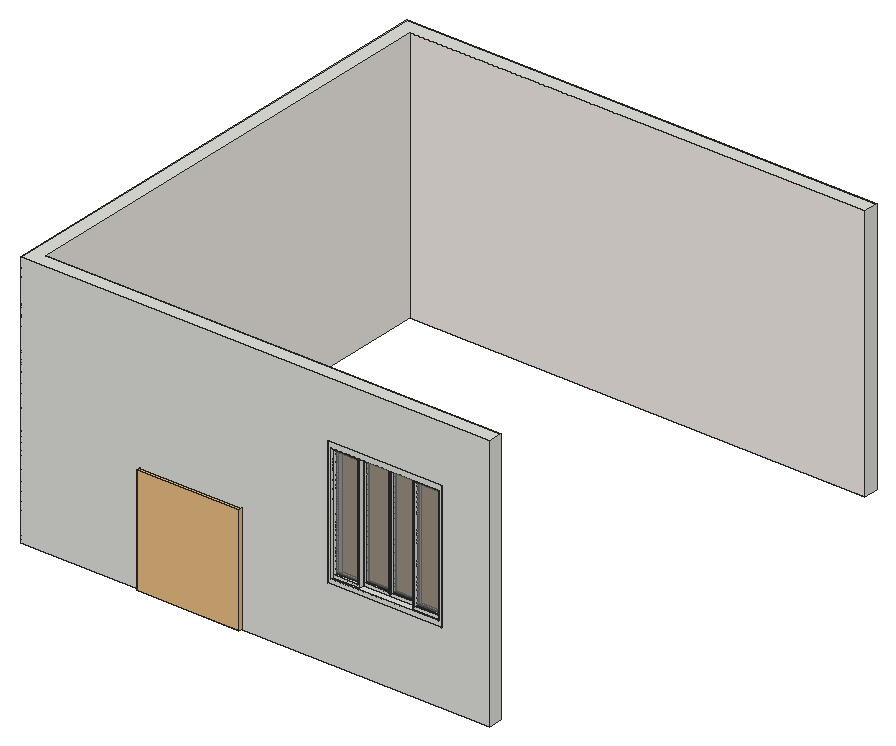
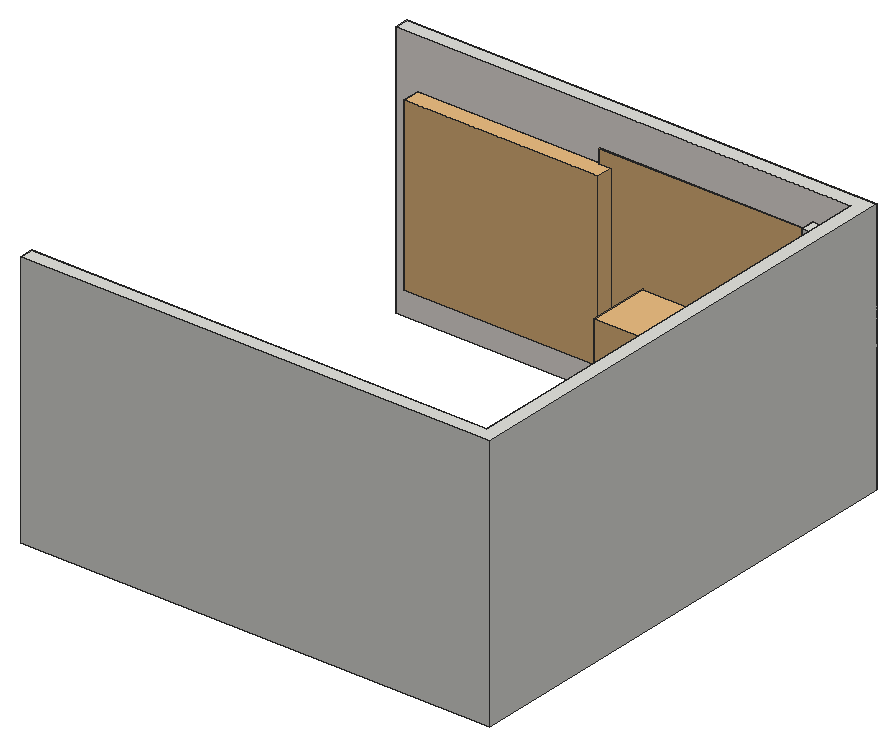
# SketchUp Ruby script. Lengths in inches.
U = 1.inch
M = Sketchup.active_model
def pt(a) = Geom::Point3d.new(a.map { |v| v * U })
def face(e, loops, mat)
  f = e.add_face(loops[0].map { |a| pt(a) })
  loops[1..].each { |l| e.add_face(l.map { |a| pt(a) }).erase! }
  f.material = f.back_material = mat if mat
  f
end
# faces: each face lists its corners as indices into pts; further lists are holes
def faces(e, pts, list, mat = nil) = list.each { |f| face(e, (f[0].is_a?(Array) ? f : [f]).map { |l| l.map { |i| pts[i] } }, mat) }
# xy, xz, yz: faces in a plane at the given z, y or x. An outline is a flat list of corners, or four numbers for a rectangle; further outlines are holes
def ring(l) = l.size == 4 ? [[l[0], l[1]], [l[2], l[1]], [l[2], l[3]], [l[0], l[3]]] : l.each_slice(2).to_a
def flat(e, list, mat, &to3) = list.each { |f| face(e, (f[0].is_a?(Array) ? f : [f]).map { |l| ring(l).map { |u, v| to3.(u, v) } }, mat) }
def xy(e, z, list, mat = nil) = flat(e, list, mat) { |x, y| [x, y, z] }
def xz(e, y, list, mat = nil) = flat(e, list, mat) { |x, z| [x, y, z] }
def yz(e, x, list, mat = nil) = flat(e, list, mat) { |y, z| [x, y, z] }
def lines(e, pts, list) = list.each { |a, b| e.add_line(pt(pts[a]), pt(pts[b])) }
# prism: a flat outline (further loops are holes) pulled along v
def prism(e, loops, v, mat = nil)
  f = face(e, loops, mat); d = Geom::Vector3d.new(v.map { |x| x * U })
  f.pushpull(f.normal.samedirection?(d) ? d.length : -d.length)
end
def box(e, o, s, mat = nil) = prism(e, [[o, [o[0] + s[0], o[1], o[2]], [o[0] + s[0], o[1] + s[1], o[2]], [o[0], o[1] + s[1], o[2]]]], [0, 0, s[2]], mat)
def at(x, y, z, deg = 0) = Geom::Transformation.translation(pt([x, y, z])) * Geom::Transformation.rotation(ORIGIN, Z_AXIS, deg.degrees)
def axes(o, x, y, z) = Geom::Transformation.new([*x, 0, *y, 0, *z, 0, *pt(o).to_a, 1])
def part(name) = M.definitions.add(name)
# library, detail: a bought-in or finely detailed component or shape, given as its bounding box
def library(name, o, s) = part(name).tap { |d| box(d.entities, o, s) }
def detail(e, o, s) = box(e.add_group.entities, o, s)
def put(e, d, t, mat = nil) = e.add_instance(d, t).tap { |i| i.material = mat if mat }
def group(e, t, mat = nil) = e.add_group.tap { |g| g.transformation = t; g.material = mat if mat }.entities
root = M.entities
M.materials.add("0001 AP 9436 AIR BREEZE").color = [243, 237, 232]
M.materials.add("Wood Floor").color = [155, 105, 61]
M.materials.add("[Carrera Marble]").color = [207, 207, 207]
M.materials.add("[Color M07]").color = [58, 58, 58]
M.materials.add("[Translucent_Glass_Gray]").color = [128, 128, 128]
M.materials["[Translucent_Glass_Gray]"].alpha = 0.5
c1 = library("wall panel",[2.24,1.65,0],[79.18,52.7,0.32])
c2 = library("Group\#53",[-10.93,-9.97,0],[57.57,44.48,60.75])
c3 = part("base")
xy(c3.entities,0,[[0,0,48,24]],"Wood Floor")
xy(c3.entities,1.5,[[[0,0,48,24],[4,4,4,20,44,20,44,4,24.12,4,24.12,5,23.88,5,23.88,4]]],"Wood Floor")
xy(c3.entities,12,[[4,4,23.88,5],[24.12,4,44,5]],"[Color M07]")
xy(c3.entities,13.5,[[4,5,44,20]])
xz(c3.entities,0,[[0,0,48,1.5]],"Wood Floor")
xz(c3.entities,4,[[4,1.5,23.88,12],[24.12,1.5,44,12]],"[Color M07]")
xz(c3.entities,5,[[23.88,1.5,24.12,12],[4,12,44,13.5]],"[Color M07]")
xz(c3.entities,20,[[4,1.5,44,13.5]],"[Color M07]")
xz(c3.entities,24,[[0,0,48,1.5]],"Wood Floor")
yz(c3.entities,0,[[0,0,24,1.5]],"Wood Floor")
yz(c3.entities,4,[[4,1.5,5,12],[5,1.5,20,13.5]],"[Color M07]")
yz(c3.entities,23.88,[[4,1.5,5,12]],"[Color M07]")
yz(c3.entities,24.12,[[4,1.5,5,12]],"[Color M07]")
yz(c3.entities,44,[[4,1.5,5,12],[5,1.5,20,13.5]],"[Color M07]")
yz(c3.entities,48,[[0,0,24,1.5]],"Wood Floor")
c4 = part("top")
xy(c4.entities,0,[[0,0,48,24]],"Wood Floor")
xy(c4.entities,0.7,[[0,0,48,18]])
xy(c4.entities,1.5,[[0,18,48,24]],"Wood Floor")
xy(c4.entities,1.5,[[0,0,48,18]],"[Carrera Marble]")
xz(c4.entities,0,[[0,0,48,0.7]],"Wood Floor")
xz(c4.entities,0,[[0,0.7,48,1.5]],"[Carrera Marble]")
xz(c4.entities,18,[[0,0.7,48,1.5]])
xz(c4.entities,24,[[0,0,48,1.5]],"Wood Floor")
yz(c4.entities,0,[[0,0,0,0.7,18,0.7,18,1.5,24,1.5,24,0]],"Wood Floor")
yz(c4.entities,0,[[0,0.7,18,1.5]],"[Carrera Marble]")
yz(c4.entities,48,[[0,0,24,0,24,1.5,18,1.5,18,0.7,0,0.7]],"Wood Floor")
yz(c4.entities,48,[[0,0.7,18,1.5]],"[Carrera Marble]")
c5 = part("centre_table")
g1 = group(c5.entities,at(0,0,0))
put(g1,c3,at(0,0,0))
put(g1,c4,at(0,0,13.5))
c6 = library("gordijn (1)",[21.44,20.39,17.56],[81.86,7.22,72])
c7 = part("Window frame")
prism(c7.entities,[[[0,70.87,0],[0,0,0],[0,0,47.24],[0,70.87,47.24]],[[0,1.97,1.97],[0,68.9,1.97],[0,68.9,45.28],[0,1.97,45.28]]],[7.875,0,0])
c8 = part("Window sash")
xy(c8.entities,0,[[0,0,3.9375,16.73]])
xy(c8.entities,0.98,[[0,0.98,1.77,15.75],[1.77,0.98,2.85,15.75],[2.85,0.98,3.9375,15.75]])
xy(c8.entities,42.32,[[0,0.98,1.77,15.75],[1.77,0.98,2.85,15.75],[2.85,0.98,3.9375,15.75]])
xy(c8.entities,43.31,[[0,0,3.9375,16.73]])
xz(c8.entities,0,[[0,0,3.9375,43.31]])
xz(c8.entities,0.98,[[0,0.98,1.77,42.32],[1.77,0.98,2.85,42.32],[2.85,0.98,3.9375,42.32]])
xz(c8.entities,15.75,[[0,0.98,1.77,42.32],[1.77,0.98,2.85,42.32],[2.85,0.98,3.9375,42.32]])
xz(c8.entities,16.73,[[0,0,3.9375,43.31]])
yz(c8.entities,0,[[[0,0,16.73,43.31],[0.98,0.98,15.75,42.32]]])
yz(c8.entities,1.77,[[0.98,0.98,15.75,42.32]],"[Translucent_Glass_Gray]")
yz(c8.entities,2.85,[[0.98,0.98,15.75,42.32]],"[Translucent_Glass_Gray]")
yz(c8.entities,3.9375,[[[0,0,16.73,43.31],[0.98,0.98,15.75,42.32]]])
c9 = part("simple window")
p = [[0,68.9,1.97],[0,35.43,1.97]]
lines(c9.entities,p,[[0,1]])
put(c9.entities,c7,at(0,0,0))
put(c9.entities,c8,axes([1.14,52.17,1.97],[0.71,0,0],[0,1,0],[0,0,1]))
put(c9.entities,c8,axes([1.14,1.97,1.97],[0.71,0,0],[0,1,0],[0,0,1]))
put(c9.entities,c8,axes([3.9375,18.7,1.97],[0.71,0,0],[0,1,0],[0,0,1]))
put(c9.entities,c8,axes([3.9375,35.43,1.97],[0.71,0,0],[0,1,0],[0,0,1]))
xy(root,0,[[0,0,0,204,198,204,198,198,6,198,6,6,198,6,198,0]])
xy(root,0.25,[[6,6,22,12]])
xy(root,30.25,[[129.72,0,177.72,6]],"0001 AP 9436 AIR BREEZE")
xy(root,84.25,[[129.72,0,177.72,6]],"0001 AP 9436 AIR BREEZE")
xy(root,96.25,[[6,6,22,12]])
xy(root,108,[[0,0,198,0,198,6,6,6,6,198,198,198,198,204,0,204]])
xz(root,0,[[[0,0,198,108],[129.72,30.25,177.72,84.25]]])
xz(root,6,[[[6,0,6,0.25,22,0.25,22,96.25,6,96.25,6,108,198,108,198,0],[129.72,30.25,177.72,84.25]]],"0001 AP 9436 AIR BREEZE")
xz(root,12,[[6,0.25,22,96.25]])
xz(root,198,[[6,0,198,108]],"0001 AP 9436 AIR BREEZE")
xz(root,204,[[0,0,198,108]])
yz(root,0,[[0,0,204,108]])
yz(root,6,[[6,0,198,0,198,108,6,108,6,96.25,12,96.25,12,0.25,6,0.25]],"0001 AP 9436 AIR BREEZE")
yz(root,22,[[6,0.25,12,96.25]])
yz(root,129.72,[[0,30.25,6,84.25]],"0001 AP 9436 AIR BREEZE")
yz(root,177.72,[[0,30.25,6,84.25]],"0001 AP 9436 AIR BREEZE")
yz(root,198,[[0,0,6,108],[198,0,204,108]])
put(root,c1,axes([114.26,6,1.12],[-1.13322,0,0],[0,0,1.68107],[0,1.8887,0]))
put(root,c2,axes([85.22,24.53,0.25],[-0.75,0,0],[0,-0.75,0],[0,0,0.75]))
put(root,c5,at(108.52,44.17,0.75,90))
put(root,c6,at(210.12,33.61,-2.62,180))
put(root,c9,axes([177.72,0,30.25],[0,0.762,0],[-0.67733,0,0],[0,0,1.143]))
